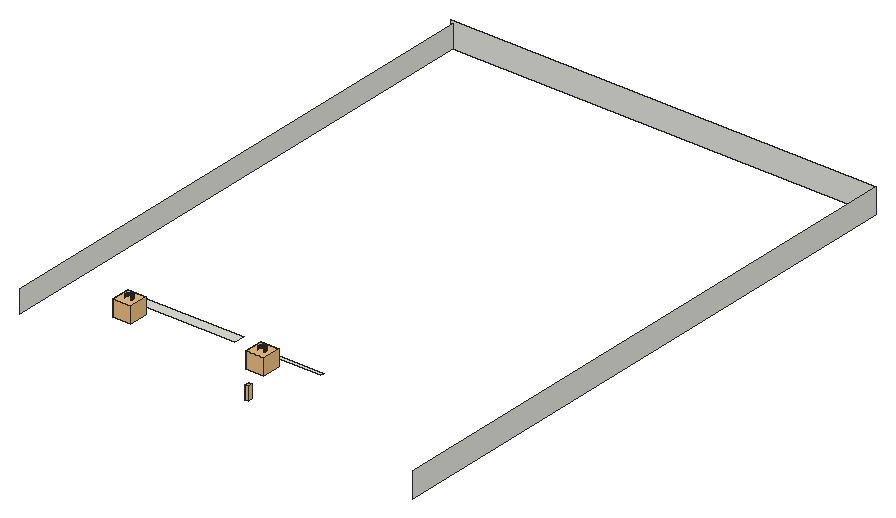
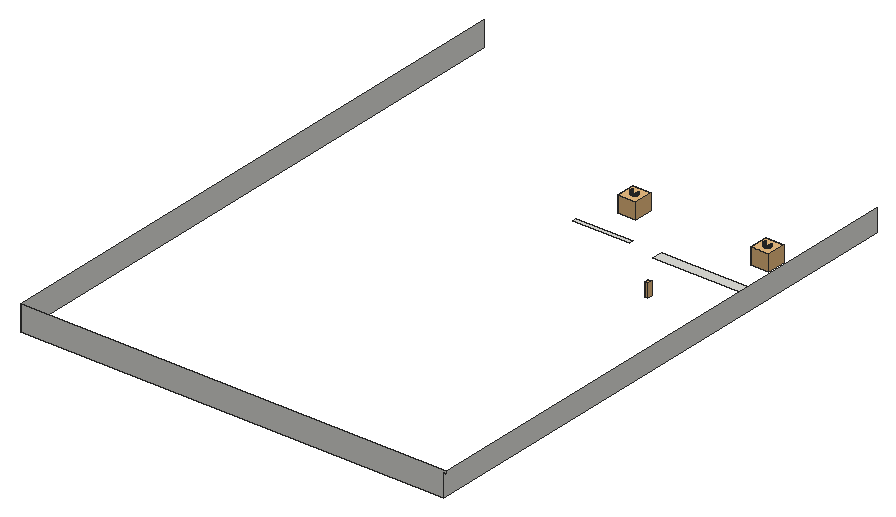
# SketchUp Ruby script. Lengths in inches.
U = 1.inch
M = Sketchup.active_model
def pt(a) = Geom::Point3d.new(a.map { |v| v * U })
def face(e, loops, mat)
  f = e.add_face(loops[0].map { |a| pt(a) })
  loops[1..].each { |l| e.add_face(l.map { |a| pt(a) }).erase! }
  f.material = f.back_material = mat if mat
  f
end
# faces: each face lists its corners as indices into pts; further lists are holes
def faces(e, pts, list, mat = nil) = list.each { |f| face(e, (f[0].is_a?(Array) ? f : [f]).map { |l| l.map { |i| pts[i] } }, mat) }
# xy, xz, yz: faces in a plane at the given z, y or x. An outline is a flat list of corners, or four numbers for a rectangle; further outlines are holes
def ring(l) = l.size == 4 ? [[l[0], l[1]], [l[2], l[1]], [l[2], l[3]], [l[0], l[3]]] : l.each_slice(2).to_a
def flat(e, list, mat, &to3) = list.each { |f| face(e, (f[0].is_a?(Array) ? f : [f]).map { |l| ring(l).map { |u, v| to3.(u, v) } }, mat) }
def xy(e, z, list, mat = nil) = flat(e, list, mat) { |x, y| [x, y, z] }
def xz(e, y, list, mat = nil) = flat(e, list, mat) { |x, z| [x, y, z] }
def yz(e, x, list, mat = nil) = flat(e, list, mat) { |y, z| [x, y, z] }
def lines(e, pts, list) = list.each { |a, b| e.add_line(pt(pts[a]), pt(pts[b])) }
# prism: a flat outline (further loops are holes) pulled along v
def prism(e, loops, v, mat = nil)
  f = face(e, loops, mat); d = Geom::Vector3d.new(v.map { |x| x * U })
  f.pushpull(f.normal.samedirection?(d) ? d.length : -d.length)
end
def box(e, o, s, mat = nil) = prism(e, [[o, [o[0] + s[0], o[1], o[2]], [o[0] + s[0], o[1] + s[1], o[2]], [o[0], o[1] + s[1], o[2]]]], [0, 0, s[2]], mat)
def at(x, y, z, deg = 0) = Geom::Transformation.translation(pt([x, y, z])) * Geom::Transformation.rotation(ORIGIN, Z_AXIS, deg.degrees)
def axes(o, x, y, z) = Geom::Transformation.new([*x, 0, *y, 0, *z, 0, *pt(o).to_a, 1])
def part(name) = M.definitions.add(name)
# library, detail: a bought-in or finely detailed component or shape, given as its bounding box
def library(name, o, s) = part(name).tap { |d| box(d.entities, o, s) }
def detail(e, o, s) = box(e.add_group.entities, o, s)
def put(e, d, t, mat = nil) = e.add_instance(d, t).tap { |i| i.material = mat if mat }
def group(e, t, mat = nil) = e.add_group.tap { |g| g.transformation = t; g.material = mat if mat }.entities
root = M.entities
M.materials.add("1122 AP 7994 PEACH ROSE").color = [254, 227, 201]
c1 = library("9",[-5.85,-5.85,-13.96],[15.28,15.28,13.96])
c2 = library("WALL LIGHT 69",[4.19,4.05,-8.78],[4.61,5.7,17.13])
xy(root,260.82,[[39,273,123,282],[147,273,195,276]])
xz(root,252,[[52.82,278.82,52.9,281.82],[52.9,278.82,52.98,281.82],[52.98,278.82,53.06,281.82],[53.06,278.82,53.14,281.82],[164.84,278.82,164.92,281.82],
  [164.92,278.82,165,281.82],[165,278.82,165.08,281.82],[165.08,278.82,165.16,281.82]],"1122 AP 7994 PEACH ROSE")
xz(root,645,[[9,278.82,9,297.82,7,297.82,7,299.82,366,299.82,366,278.82]])
yz(root,9,[[189,278.82,645,297.82]])
yz(root,49.98,[[248.92,278.82,249,281.82],[249,278.82,249.08,281.82]],"1122 AP 7994 PEACH ROSE")
yz(root,49.99,[[248.76,278.82,248.84,281.82],[249.16,278.82,249.24,281.82]],"1122 AP 7994 PEACH ROSE")
yz(root,55.96,[[248.61,278.82,248.6875,281.82],[249.3125,278.82,249.39,281.82]],"1122 AP 7994 PEACH ROSE")
yz(root,55.98,[[248.84,278.82,248.92,281.82],[248.92,278.82,249,281.82],[249,278.82,249.08,281.82],[249.08,278.82,249.16,281.82]],"1122 AP 7994 PEACH ROSE")
yz(root,162,[[248.84,278.82,248.92,281.82],[248.92,278.82,249,281.82],[249,278.82,249.08,281.82],[249.08,278.82,249.16,281.82]],"1122 AP 7994 PEACH ROSE")
yz(root,168,[[248.84,278.82,248.92,281.82],[248.92,278.82,249,281.82],[249,278.82,249.08,281.82],[249.08,278.82,249.16,281.82]],"1122 AP 7994 PEACH ROSE")
yz(root,366,[[156,278.82,645,299.82]])
p = [[167.64,247.57,278.82],[167.6,247.5,278.82],[167.6,247.5,281.82],[167.64,247.57,281.82],[50.34,247.57,278.82],[50.31,247.64,278.82],
  [50.31,247.64,281.82],[50.34,247.57,281.82],[50.27,247.71,278.82],[50.27,247.71,281.82],[55.65,247.64,278.82],[55.62,247.57,278.82],
  [55.62,247.57,281.82],[55.65,247.64,281.82],[55.6875,247.71,278.82],[55.6875,247.71,281.82],[162.36,247.57,278.82],[162.33,247.64,278.82],
  [162.33,247.64,281.82],[162.36,247.57,281.82],[162.29,247.71,278.82],[162.29,247.71,281.82],[167.67,247.64,278.82],[167.67,247.64,281.82],
  [167.71,247.71,278.82],[167.71,247.71,281.82],[50.24,247.78,278.82],[50.24,247.78,281.82],[55.72,247.78,278.82],[55.72,247.78,281.82],
  [162.26,247.78,278.82],[162.26,247.78,281.82],[167.74,247.78,278.82],[167.74,247.78,281.82],[50.21,247.85,278.82],[50.21,247.85,281.82],
  [55.75,247.85,278.82],[55.75,247.85,281.82],[162.23,247.85,278.82],[162.23,247.85,281.82],[167.77,247.85,278.82],[167.77,247.85,281.82],
  [50.18,247.92,278.82],[50.18,247.92,281.82],[50.15,248,278.82],[50.15,248,281.82],[55.78,247.92,278.82],[55.78,247.92,281.82],
  [55.81,248,278.82],[55.81,248,281.82],[162.2,247.92,278.82],[162.2,247.92,281.82],[162.17,248,278.82],[162.17,248,281.82],
  [167.8,247.92,278.82],[167.8,247.92,281.82],[167.83,248,278.82],[167.83,248,281.82],[50.13,248.07,278.82],[50.13,248.07,281.82],
  [55.83,248.07,278.82],[55.83,248.07,281.82],[162.15,248.07,278.82],[162.15,248.07,281.82],[167.85,248.07,278.82],[167.85,248.07,281.82],
  [50.1,248.15,278.82],[50.1,248.15,281.82],[50.08,248.22,278.82],[50.08,248.22,281.82],[55.86,248.15,278.82],[55.86,248.15,281.82],
  [55.88,248.22,278.82],[55.88,248.22,281.82],[162.125,248.15,278.82],[162.125,248.15,281.82],[162.1,248.22,278.82],[162.1,248.22,281.82],
  [167.875,248.15,278.82],[167.875,248.15,281.82],[167.9,248.22,278.82],[167.9,248.22,281.82],[50.0625,248.3,278.82],[50.0625,248.3,281.82],
  [55.9,248.3,278.82],[55.9,248.3,281.82],[162.08,248.3,278.82],[162.08,248.3,281.82],[167.92,248.3,278.82],[167.92,248.3,281.82],
  [50.05,248.375,278.82],[50.05,248.375,281.82],[55.92,248.375,278.82],[55.92,248.375,281.82],[162.07,248.375,278.82],[162.07,248.375,281.82],
  [167.93,248.375,278.82],[167.93,248.375,281.82],[50.03,248.45,278.82],[50.03,248.45,281.82],[55.93,248.45,278.82],[55.93,248.45,281.82],
  [162.05,248.45,278.82],[162.05,248.45,281.82],[167.95,248.45,278.82],[167.95,248.45,281.82],[50.02,248.53,278.82],[50.02,248.53,281.82],
  [50.01,248.61,278.82],[50.01,248.61,281.82],[55.94,248.53,278.82],[55.94,248.53,281.82],[55.96,248.61,278.82],[55.96,248.61,281.82],
  [162.04,248.53,278.82],[162.04,248.53,281.82],[162.03,248.61,278.82],[162.03,248.61,281.82],[167.96,248.53,278.82],[167.96,248.53,281.82],
  [167.97,248.61,278.82],[167.97,248.61,281.82],[50,248.6875,278.82],[50,248.6875,281.82],[162.02,248.6875,278.82],[162.02,248.6875,281.82],
  [167.98,248.6875,278.82],[167.98,248.6875,281.82],[49.99,248.76,278.82],[49.99,248.76,281.82],[55.97,248.76,278.82],[55.96,248.6875,278.82],
  [55.96,248.6875,281.82],[55.97,248.76,281.82],[162.01,248.76,278.82],[162.01,248.76,281.82],[167.99,248.76,278.82],[167.99,248.76,281.82],
  [49.99,248.84,278.82],[49.98,248.92,278.82],[49.98,248.92,281.82],[49.99,248.84,281.82],[55.98,248.84,278.82],[55.98,248.84,281.82],
  [162,248.84,278.82],[162,248.84,281.82],[168,248.84,278.82],[168,248.84,281.82],[49.98,249.08,278.82],[49.99,249.16,278.82],
  [49.99,249.16,281.82],[49.98,249.08,281.82],[49.99,249.24,278.82],[50,249.3125,278.82],[50,249.3125,281.82],[49.99,249.24,281.82],
  [55.97,249.24,278.82],[55.98,249.16,278.82],[55.98,249.16,281.82],[55.97,249.24,281.82],[55.96,249.3125,278.82],[55.96,249.3125,281.82],
  [162,249.16,278.82],[162.01,249.24,278.82],[162.01,249.24,281.82],[162,249.16,281.82],[162.02,249.3125,278.82],[162.02,249.3125,281.82],
  [167.99,249.24,278.82],[168,249.16,278.82],[168,249.16,281.82],[167.99,249.24,281.82],[167.98,249.3125,278.82],[167.98,249.3125,281.82],
  [50.01,249.39,278.82],[50.01,249.39,281.82],[162.03,249.39,278.82],[162.03,249.39,281.82],[167.97,249.39,278.82],[167.97,249.39,281.82],
  [50.02,249.47,278.82],[50.02,249.47,281.82],[55.94,249.47,278.82],[55.96,249.39,278.82],[55.96,249.39,281.82],[55.94,249.47,281.82],
  [162.04,249.47,278.82],[162.04,249.47,281.82],[167.96,249.47,278.82],[167.96,249.47,281.82],[50.03,249.55,278.82],[50.03,249.55,281.82],
  [50.05,249.625,278.82],[50.05,249.625,281.82],[55.93,249.55,278.82],[55.93,249.55,281.82],[55.92,249.625,278.82],[55.92,249.625,281.82],
  [162.05,249.55,278.82],[162.05,249.55,281.82],[162.07,249.625,278.82],[162.07,249.625,281.82],[167.95,249.55,278.82],[167.95,249.55,281.82],
  [167.93,249.625,278.82],[167.93,249.625,281.82],[50.0625,249.7,278.82],[50.0625,249.7,281.82],[55.9,249.7,278.82],[55.9,249.7,281.82],
  [162.08,249.7,278.82],[162.08,249.7,281.82],[167.92,249.7,278.82],[167.92,249.7,281.82],[50.08,249.78,278.82],[50.08,249.78,281.82],
  [55.88,249.78,278.82],[55.88,249.78,281.82],[162.1,249.78,278.82],[162.1,249.78,281.82],[167.9,249.78,278.82],[167.9,249.78,281.82],
  [50.1,249.85,278.82],[50.1,249.85,281.82],[55.86,249.85,278.82],[55.86,249.85,281.82],[162.125,249.85,278.82],[162.125,249.85,281.82],
  [167.875,249.85,278.82],[167.875,249.85,281.82],[50.13,249.93,278.82],[50.13,249.93,281.82],[50.15,250,278.82],[50.15,250,281.82],
  [55.83,249.93,278.82],[55.83,249.93,281.82],[55.81,250,278.82],[55.81,250,281.82],[162.15,249.93,278.82],[162.15,249.93,281.82],
  [162.17,250,278.82],[162.17,250,281.82],[167.83,250,278.82],[167.85,249.93,278.82],[167.85,249.93,281.82],[167.83,250,281.82],
  [50.18,250.08,278.82],[50.18,250.08,281.82],[55.78,250.08,278.82],[55.78,250.08,281.82],[162.2,250.08,278.82],[162.2,250.08,281.82],
  [167.8,250.08,278.82],[167.8,250.08,281.82],[50.21,250.15,278.82],[50.21,250.15,281.82],[50.24,250.22,278.82],[50.24,250.22,281.82],
  [55.72,250.22,278.82],[55.75,250.15,278.82],[55.75,250.15,281.82],[55.72,250.22,281.82],[162.23,250.15,278.82],[162.23,250.15,281.82],
  [162.26,250.22,278.82],[162.26,250.22,281.82],[167.74,250.22,278.82],[167.77,250.15,278.82],[167.77,250.15,281.82],[167.74,250.22,281.82],
  [50.27,250.29,278.82],[50.27,250.29,281.82],[55.6875,250.29,278.82],[55.6875,250.29,281.82],[162.29,250.29,278.82],[162.29,250.29,281.82],
  [167.71,250.29,278.82],[167.71,250.29,281.82],[50.31,250.36,278.82],[50.31,250.36,281.82],[55.65,250.36,278.82],[55.65,250.36,281.82],
  [162.33,250.36,278.82],[162.33,250.36,281.82],[167.67,250.36,278.82],[167.67,250.36,281.82],[50.34,250.43,278.82],[50.34,250.43,281.82],
  [50.38,250.5,278.82],[50.38,250.5,281.82],[55.62,250.43,278.82],[55.62,250.43,281.82],[55.58,250.5,278.82],[55.58,250.5,281.82],
  [162.36,250.43,278.82],[162.36,250.43,281.82],[162.4,250.5,278.82],[162.4,250.5,281.82],[167.64,250.43,278.82],[167.64,250.43,281.82],
  [167.6,250.5,278.82],[167.6,250.5,281.82],[50.42,250.57,278.82],[50.42,250.57,281.82],[55.54,250.57,278.82],[55.54,250.57,281.82],
  [162.44,250.57,278.82],[162.44,250.57,281.82],[167.56,250.57,278.82],[167.56,250.57,281.82],[50.46,250.63,278.82],[50.46,250.63,281.82],
  [50.51,250.7,278.82],[50.51,250.7,281.82],[55.5,250.63,278.82],[55.5,250.63,281.82],[55.45,250.7,278.82],[55.45,250.7,281.82],
  [162.48,250.63,278.82],[162.48,250.63,281.82],[162.53,250.7,278.82],[162.53,250.7,281.82],[167.52,250.63,278.82],[167.52,250.63,281.82],
  [167.47,250.7,278.82],[167.47,250.7,281.82],[50.55,250.76,278.82],[50.55,250.76,281.82],[55.41,250.76,278.82],[55.41,250.76,281.82],
  [162.57,250.76,278.82],[162.57,250.76,281.82],[167.43,250.76,278.82],[167.43,250.76,281.82],[50.6,250.83,278.82],[50.6,250.83,281.82],
  [50.65,250.89,278.82],[50.65,250.89,281.82],[55.3125,250.89,278.82],[55.36,250.83,278.82],[55.36,250.83,281.82],[55.3125,250.89,281.82],
  [162.62,250.83,278.82],[162.62,250.83,281.82],[162.67,250.89,278.82],[162.67,250.89,281.82],[167.33,250.89,278.82],[167.38,250.83,278.82],
  [167.38,250.83,281.82],[167.33,250.89,281.82],[50.7,250.95,278.82],[50.7,250.95,281.82],[50.75,251.01,278.82],[50.75,251.01,281.82],
  [55.21,251.01,278.82],[55.26,250.95,278.82],[55.26,250.95,281.82],[55.21,251.01,281.82],[162.72,250.95,278.82],[162.72,250.95,281.82],
  [162.77,251.01,278.82],[162.77,251.01,281.82],[167.23,251.01,278.82],[167.28,250.95,278.82],[167.28,250.95,281.82],[167.23,251.01,281.82],
  [50.8,251.07,278.82],[50.8,251.07,281.82],[55.16,251.07,278.82],[55.16,251.07,281.82],[162.82,251.07,278.82],[162.82,251.07,281.82],
  [167.18,251.07,278.82],[167.18,251.07,281.82],[50.86,251.12,278.82],[50.86,251.12,281.82],[50.92,251.18,278.82],[50.92,251.18,281.82],
  [55.05,251.18,278.82],[55.1,251.12,278.82],[55.1,251.12,281.82],[55.05,251.18,281.82],[162.88,251.12,278.82],[162.88,251.12,281.82],
  [162.93,251.18,278.82],[162.93,251.18,281.82],[167.12,251.12,278.82],[167.12,251.12,281.82],[167.07,251.18,278.82],[167.07,251.18,281.82],
  [50.97,251.23,278.82],[50.97,251.23,281.82],[51.03,251.28,278.82],[51.03,251.28,281.82],[54.93,251.28,278.82],[54.99,251.23,278.82],
  [54.99,251.23,281.82],[54.93,251.28,281.82],[162.99,251.23,278.82],[162.99,251.23,281.82],[163.05,251.28,278.82],[163.05,251.28,281.82],
  [166.95,251.28,278.82],[167.01,251.23,278.82],[167.01,251.23,281.82],[166.95,251.28,281.82],[51.09,251.33,278.82],[51.09,251.33,281.82],
  [51.15,251.38,278.82],[51.15,251.38,281.82],[54.81,251.38,278.82],[54.87,251.33,278.82],[54.87,251.33,281.82],[54.81,251.38,281.82],
  [163.11,251.33,278.82],[163.11,251.33,281.82],[163.17,251.38,278.82],[163.17,251.38,281.82],[166.83,251.38,278.82],[166.89,251.33,278.82],
  [166.89,251.33,281.82],[166.83,251.38,281.82],[51.22,251.43,278.82],[51.22,251.43,281.82],[51.28,251.47,278.82],[51.28,251.47,281.82],
  [54.74,251.43,278.82],[54.74,251.43,281.82],[54.68,251.47,278.82],[54.68,251.47,281.82],[163.24,251.43,278.82],[163.24,251.43,281.82],
  [163.3,251.47,278.82],[163.3,251.47,281.82],[166.7,251.47,278.82],[166.76,251.43,278.82],[166.76,251.43,281.82],[166.7,251.47,281.82],
  [51.35,251.52,278.82],[51.35,251.52,281.82],[51.41,251.56,278.82],[51.41,251.56,281.82],[54.55,251.56,278.82],[54.61,251.52,278.82],
  [54.61,251.52,281.82],[54.55,251.56,281.82],[163.37,251.52,278.82],[163.37,251.52,281.82],[163.43,251.56,278.82],[163.43,251.56,281.82],
  [166.63,251.52,278.82],[166.63,251.52,281.82],[166.57,251.56,278.82],[166.57,251.56,281.82],[51.48,251.6,278.82],[51.48,251.6,281.82],
  [51.55,251.64,278.82],[51.55,251.64,281.82],[51.62,251.67,278.82],[51.62,251.67,281.82],[54.34,251.67,278.82],[54.41,251.64,278.82],
  [54.41,251.64,281.82],[54.34,251.67,281.82],[54.48,251.6,278.82],[54.48,251.6,281.82],[163.5,251.6,278.82],[163.5,251.6,281.82],
  [163.57,251.64,278.82],[163.57,251.64,281.82],[163.64,251.67,278.82],[163.64,251.67,281.82],[166.43,251.64,278.82],[166.5,251.6,278.82],
  [166.5,251.6,281.82],[166.43,251.64,281.82],[166.36,251.67,278.82],[166.36,251.67,281.82],[51.6875,251.71,278.82],[51.6875,251.71,281.82],
  [51.76,251.74,278.82],[51.76,251.74,281.82],[51.83,251.77,278.82],[51.83,251.77,281.82],[54.13,251.77,278.82],[54.2,251.74,278.82],
  [54.2,251.74,281.82],[54.13,251.77,281.82],[54.27,251.71,278.82],[54.27,251.71,281.82],[163.71,251.71,278.82],[163.71,251.71,281.82],
  [163.78,251.74,278.82],[163.78,251.74,281.82],[163.85,251.77,278.82],[163.85,251.77,281.82],[166.15,251.77,278.82],[166.22,251.74,278.82],
  [166.22,251.74,281.82],[166.15,251.77,281.82],[166.29,251.71,278.82],[166.29,251.71,281.82],[51.91,251.8,278.82],[51.91,251.8,281.82],
  [51.98,251.83,278.82],[51.98,251.83,281.82],[52.05,251.85,278.82],[52.05,251.85,281.82],[53.91,251.85,278.82],[53.98,251.83,278.82],
  [53.98,251.83,281.82],[53.91,251.85,281.82],[54.06,251.8,278.82],[54.06,251.8,281.82],[163.92,251.8,278.82],[163.92,251.8,281.82],
  [164,251.83,278.82],[164,251.83,281.82],[164.07,251.85,278.82],[164.07,251.85,281.82],[165.93,251.85,278.82],[166,251.83,278.82],
  [166,251.83,281.82],[165.93,251.85,281.82],[166.08,251.8,278.82],[166.08,251.8,281.82],[52.13,251.875,278.82],[52.13,251.875,281.82],
  [52.2,251.9,278.82],[52.2,251.9,281.82],[52.28,251.92,278.82],[52.28,251.92,281.82],[52.36,251.93,278.82],[52.36,251.93,281.82],
  [52.43,251.95,278.82],[52.43,251.95,281.82],[52.51,251.96,278.82],[52.51,251.96,281.82],[53.53,251.95,278.82],[53.6,251.93,278.82],
  [53.6,251.93,281.82],[53.53,251.95,281.82],[53.45,251.96,278.82],[53.45,251.96,281.82],[53.68,251.92,278.82],[53.68,251.92,281.82],
  [53.76,251.9,278.82],[53.76,251.9,281.82],[53.83,251.875,278.82],[53.83,251.875,281.82],[164.15,251.875,278.82],[164.15,251.875,281.82],
  [164.22,251.9,278.82],[164.22,251.9,281.82],[164.3,251.92,278.82],[164.3,251.92,281.82],[164.375,251.93,278.82],[164.375,251.93,281.82],
  [164.45,251.95,278.82],[164.45,251.95,281.82],[164.53,251.96,278.82],[164.53,251.96,281.82],[165.55,251.95,278.82],[165.625,251.93,278.82],
  [165.625,251.93,281.82],[165.55,251.95,281.82],[165.47,251.96,278.82],[165.47,251.96,281.82],[165.7,251.92,278.82],[165.7,251.92,281.82],
  [165.78,251.9,278.82],[165.78,251.9,281.82],[165.85,251.875,278.82],[165.85,251.875,281.82],[52.59,251.97,278.82],[52.59,251.97,281.82],
  [52.67,251.98,278.82],[52.67,251.98,281.82],[52.75,251.99,278.82],[52.75,251.99,281.82],[52.82,252,278.82],[52.82,252,281.82],
  [53.14,252,278.82],[53.22,251.99,278.82],[53.22,251.99,281.82],[53.14,252,281.82],[53.29,251.98,278.82],[53.29,251.98,281.82],
  [53.37,251.97,278.82],[53.37,251.97,281.82],[164.61,251.97,278.82],[164.61,251.97,281.82],[164.6875,251.98,278.82],[164.6875,251.98,281.82],
  [164.76,251.99,278.82],[164.76,251.99,281.82],[164.84,252,278.82],[164.84,252,281.82],[165.24,251.99,278.82],[165.3125,251.98,278.82],
  [165.3125,251.98,281.82],[165.24,251.99,281.82],[165.16,252,278.82],[165.16,252,281.82],[165.39,251.97,278.82],[165.39,251.97,281.82]]
faces(root,p,[[0,1,2,3],[4,5,6,7],[5,8,9,6],[10,11,12,13],[14,10,13,15],[16,17,18,19],[17,20,21,18],[22,0,3,23],
  [24,22,23,25],[8,26,27,9],[28,14,15,29],[20,30,31,21],[32,24,25,33],[26,34,35,27],[36,28,29,37],[30,38,39,31],
  [40,32,33,41],[34,42,43,35],[42,44,45,43],[46,36,37,47],[48,46,47,49],[38,50,51,39],[50,52,53,51],[54,40,41,55],
  [56,54,55,57],[44,58,59,45],[60,48,49,61],[52,62,63,53],[64,56,57,65],[58,66,67,59],[66,68,69,67],[70,60,61,71],
  [72,70,71,73],[62,74,75,63],[74,76,77,75],[78,64,65,79],[80,78,79,81],[68,82,83,69],[84,72,73,85],[76,86,87,77],
  [88,80,81,89],[82,90,91,83],[92,84,85,93],[86,94,95,87],[96,88,89,97],[90,98,99,91],[100,92,93,101],[94,102,103,95],
  [104,96,97,105],[98,106,107,99],[106,108,109,107],[110,100,101,111],[112,110,111,113],[102,114,115,103],[114,116,117,115],[118,104,105,119],
  [120,118,119,121],[108,122,123,109],[116,124,125,117],[126,120,121,127],[122,128,129,123],[130,131,132,133],[124,134,135,125],[136,126,127,137],
  [138,139,140,141],[142,130,133,143],[134,144,145,135],[146,136,137,147],[148,149,150,151],[152,153,154,155],[156,157,158,159],[160,156,159,161],
  [162,163,164,165],[163,166,167,164],[168,169,170,171],[172,168,171,173],[153,174,175,154],[166,176,177,167],[178,172,173,179],[174,180,181,175],
  [182,183,184,185],[176,186,187,177],[188,178,179,189],[180,190,191,181],[190,192,193,191],[194,182,185,195],[196,194,195,197],[186,198,199,187],
  [198,200,201,199],[202,188,189,203],[204,202,203,205],[192,206,207,193],[208,196,197,209],[200,210,211,201],[212,204,205,213],[206,214,215,207],
  [216,208,209,217],[210,218,219,211],[220,212,213,221],[214,222,223,215],[224,216,217,225],[218,226,227,219],[228,220,221,229],[222,230,231,223],
  [230,232,233,231],[234,224,225,235],[236,234,235,237],[226,238,239,227],[238,240,241,239],[242,243,244,245],[243,228,229,244],[232,246,247,233],
  [248,236,237,249],[240,250,251,241],[252,242,245,253],[246,254,255,247],[254,256,257,255],[258,259,260,261],[259,248,249,260],[250,262,263,251],
  [262,264,265,263],[266,267,268,269],[267,252,253,268],[256,270,271,257],[272,258,261,273],[264,274,275,265],[276,266,269,277],[270,278,279,271],
  [280,272,273,281],[274,282,283,275],[284,276,277,285],[278,286,287,279],[286,288,289,287],[290,280,281,291],[292,290,291,293],[282,294,295,283],
  [294,296,297,295],[298,284,285,299],[300,298,299,301],[288,302,303,289],[304,292,293,305],[296,306,307,297],[308,300,301,309],[302,310,311,303],
  [310,312,313,311],[314,304,305,315],[316,314,315,317],[306,318,319,307],[318,320,321,319],[322,308,309,323],[324,322,323,325],[312,326,327,313],
  [328,316,317,329],[320,330,331,321],[332,324,325,333],[326,334,335,327],[334,336,337,335],[338,339,340,341],[339,328,329,340],[330,342,343,331],
  [342,344,345,343],[346,347,348,349],[347,332,333,348],[336,350,351,337],[350,352,353,351],[354,355,356,357],[355,338,341,356],[344,358,359,345],
  [358,360,361,359],[362,363,364,365],[363,346,349,364],[352,366,367,353],[368,354,357,369],[360,370,371,361],[372,362,365,373],[366,374,375,367],
  [374,376,377,375],[378,379,380,381],[379,368,369,380],[370,382,383,371],[382,384,385,383],[386,372,373,387],[388,386,387,389],[376,390,391,377],
  [390,392,393,391],[394,395,396,397],[395,378,381,396],[384,398,399,385],[398,400,401,399],[402,403,404,405],[403,388,389,404],[392,406,407,393],
  [406,408,409,407],[410,411,412,413],[411,394,397,412],[400,414,415,401],[414,416,417,415],[418,419,420,421],[419,402,405,420],[408,422,423,409],
  [422,424,425,423],[426,410,413,427],[428,426,427,429],[416,430,431,417],[430,432,433,431],[434,435,436,437],[435,418,421,436],[424,438,439,425],
  [438,440,441,439],[442,443,444,445],[443,428,429,444],[432,446,447,433],[446,448,449,447],[450,434,437,451],[452,450,451,453],[440,454,455,441],
  [454,456,457,455],[456,458,459,457],[460,461,462,463],[461,464,465,462],[464,442,445,465],[448,466,467,449],[466,468,469,467],[468,470,471,469],
  [472,473,474,475],[476,472,475,477],[473,452,453,474],[458,478,479,459],[478,480,481,479],[480,482,483,481],[484,485,486,487],[485,488,489,486],
  [488,460,463,489],[470,490,491,471],[490,492,493,491],[492,494,495,493],[496,497,498,499],[497,500,501,498],[500,476,477,501],[482,502,503,483],
  [502,504,505,503],[504,506,507,505],[508,509,510,511],[509,512,513,510],[512,484,487,513],[494,514,515,495],[514,516,517,515],[516,518,519,517],
  [520,521,522,523],[521,524,525,522],[524,496,499,525],[506,526,527,507],[526,528,529,527],[528,530,531,529],[530,532,533,531],[532,534,535,533],
  [534,536,537,535],[538,539,540,541],[542,538,541,543],[539,544,545,540],[544,546,547,545],[548,508,511,549],[546,548,549,547],[518,550,551,519],
  [550,552,553,551],[552,554,555,553],[554,556,557,555],[556,558,559,557],[558,560,561,559],[562,563,564,565],[566,562,565,567],[563,568,569,564],
  [568,570,571,569],[570,572,573,571],[572,520,523,573],[536,574,575,537],[574,576,577,575],[576,578,579,577],[578,580,581,579],[582,583,584,585],
  [583,586,587,584],[586,588,589,587],[588,542,543,589],[560,590,591,561],[590,592,593,591],[592,594,595,593],[594,596,597,595],[598,599,600,601],
  [602,598,601,603],[599,604,605,600],[604,566,567,605]],"1122 AP 7994 PEACH ROSE")
put(root,c1,at(163.21,247.21,280.07))
put(root,c1,at(51.19,247.21,280.07))
put(root,c2,axes([131.375,266.66,228.42],[0.65,0,0],[0,0.65,0],[0,0,0.65]))
